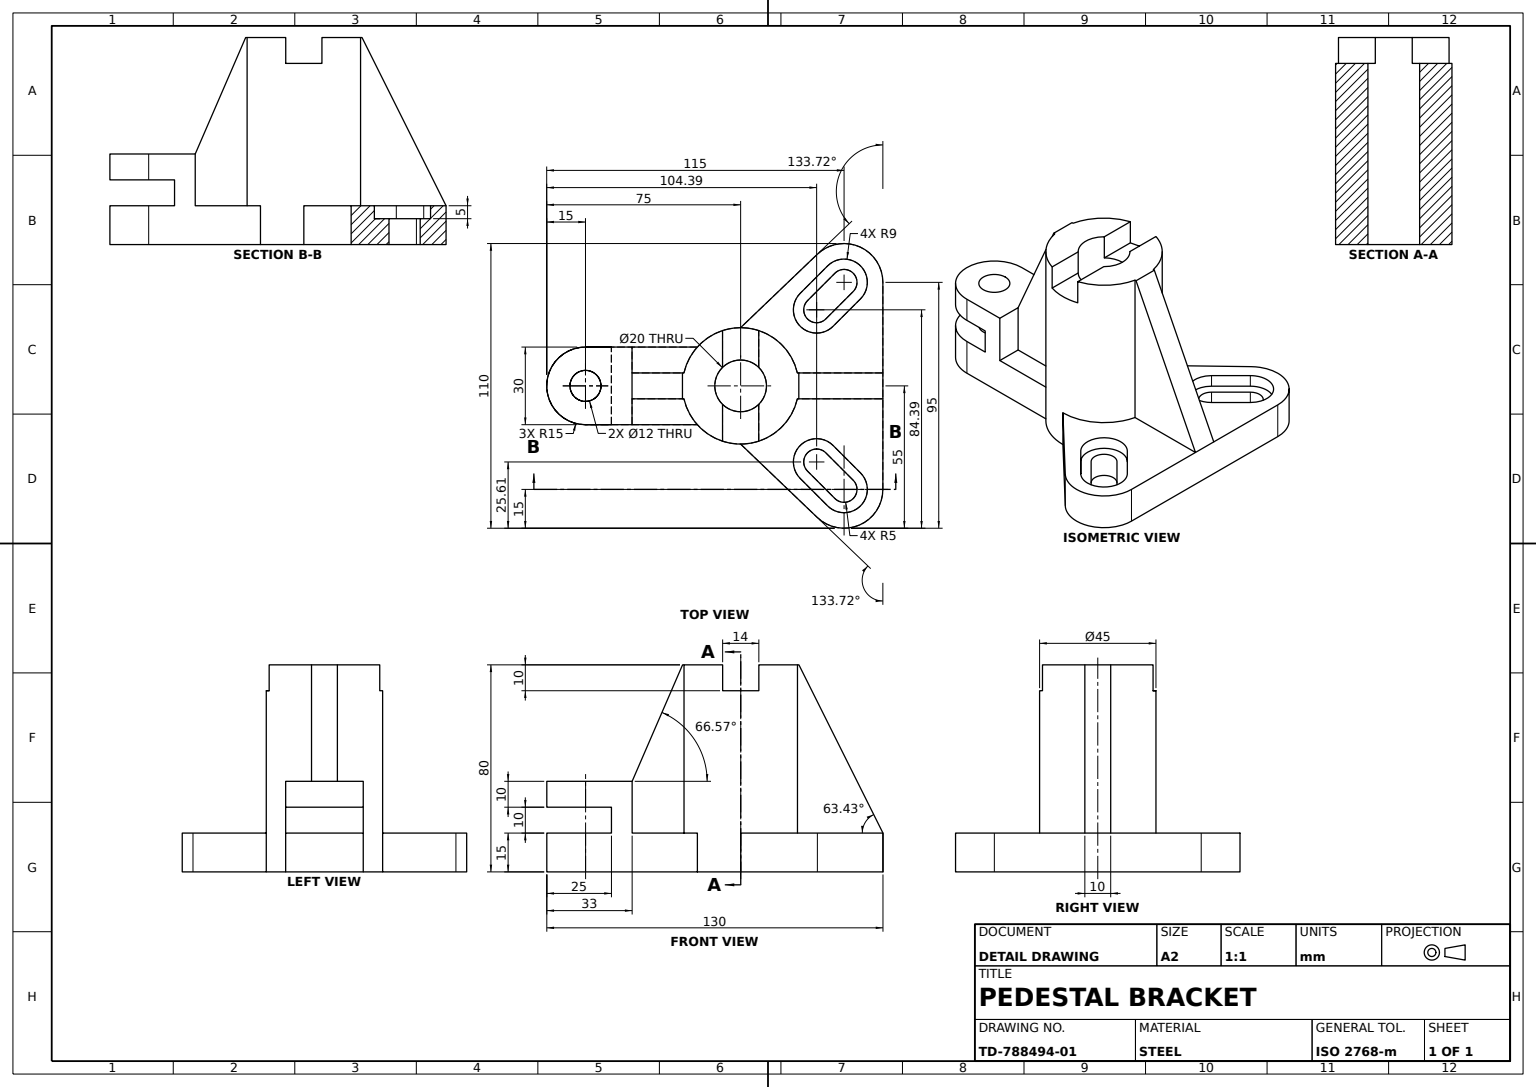
solid
v1 (-60,15,-6)
v2 (-60,15,6)
e1 v1 v2 CIRCLE(AX(P(-60,15,0),D(0,-1,0),D(0,0,-1)),6)
e2 v2 v1 CIRCLE(AX(P(-60,15,0),D(0,-1,0),D(0,0,-1)),6)
v3 (-60,15,15)
v4 (-60,15,-15)
e3 v3 v4 CIRCLE(AX(P(-60,15,0),D(0,-1,0),D(0,0,-1)),15)
v5 (-50,15,15)
e4 v5 v3 LINE
v6 (-50,15,-15)
e5 v5 v6 LINE
e6 v4 v6 LINE
face PLANE(AX(P(-75,15,15),D(0,-1,0),D(0,0,-1))) rev [e1 e2] [-e3 -e4 e5 -e6]
v7 (29.632367,15,-50.840304)
v8 (0,15,-22.5)
e7 v7 v8 LINE
v9 (29.632367,0,-50.840304)
e8 v7 v9 LINE
v10 (0,0,-22.5)
e9 v9 v10 LINE
e10 v8 v10 LINE
face PLANE(AX(P(-11.238829,15,-11.751219),D(0.691175529,0,0.722686923),D(0.722686923,0,-0.691175529))) rev [-e7 e8 e9 -e10]
v11 (36.464466,10,43.535534)
v12 (36.464466,0,43.535534)
e11 v11 v12 LINE
v13 (25.857864,0,32.928932)
e12 v12 v13 LINE
v14 (25.857864,10,32.928932)
e13 v14 v13 LINE
e14 v11 v14 LINE
face PLANE(AX(P(36.464466,80,43.535534),D(0.707106781,0,-0.707106781),D(-0.707106781,0,-0.707106781))) [e11 e12 -e13 -e14]
v15 (-42,35,-5)
v16 (-42,35,-15)
e15 v15 v16 LINE
v17 (-60,35,-15)
e16 v16 v17 LINE
v18 (-60,35,15)
e17 v17 v18 CIRCLE(AX(P(-60,35,0),D(0,1,0),D(0,0,1)),15)
v19 (-42,35,15)
e18 v18 v19 LINE
v20 (-42,35,5)
e19 v19 v20 LINE
e20 v15 v20 LINE
v21 (-60,35,6)
v22 (-60,35,-6)
e21 v21 v22 CIRCLE(AX(P(-60,35,0),D(0,1,0),D(0,0,1)),6)
e22 v22 v21 CIRCLE(AX(P(-60,35,0),D(0,1,0),D(0,0,1)),6)
face PLANE(AX(P(-60,35,0),D(0,1,0),D(0,0,1))) [e15 e16 e17 e18 e19 -e20] [-e21 -e22]
v23 (-16.77051,15,-15)
v24 (-21.937411,15,-5)
e23 v23 v24 CIRCLE(AX(P(0,15,0),D(0,1,0),D(0,0,1)),22.5)
v25 (-42,15,-15)
e24 v25 v23 LINE
v26 (-42,15,-5)
e25 v26 v25 LINE
e26 v26 v24 LINE
face PLANE(AX(P(0,15,0),D(0,1,0),D(0,0,1))) [-e23 -e24 -e25 e26]
v27 (-42,15,15)
v28 (-42,15,5)
e27 v27 v28 LINE
v29 (-16.77051,15,15)
e28 v27 v29 LINE
v30 (-21.937411,15,5)
e29 v30 v29 CIRCLE(AX(P(0,15,0),D(0,1,0),D(0,0,1)),22.5)
e30 v28 v30 LINE
face PLANE(AX(P(0,15,0),D(0,1,0),D(0,0,1))) [-e27 e28 -e29 -e30]
v31 (-21.937411,80,5)
v32 (-7,80,21.383405)
e31 v31 v32 CIRCLE(AX(P(0,80,0),D(0,1,0),D(0,0,1)),22.5)
e32 v31 v30 LINE
v33 (-16.77051,0,15)
e33 v29 v33 LINE
v34 (0,0,22.5)
e34 v33 v34 CIRCLE(AX(P(0,0,0),D(0,1,0),D(0,0,1)),22.5)
v35 (0,15,22.5)
e35 v35 v34 LINE
v36 (21.937411,15,5)
e36 v35 v36 CIRCLE(AX(P(0,15,0),D(0,1,0),D(0,0,1)),22.5)
v37 (21.937411,80,5)
e37 v36 v37 LINE
v38 (7,80,21.383405)
e38 v38 v37 CIRCLE(AX(P(0,80,0),D(0,1,0),D(0,0,1)),22.5)
v39 (7,70,21.383405)
e39 v38 v39 LINE
v40 (-7,70,21.383405)
e40 v40 v39 CIRCLE(AX(P(0,70,0),D(0,1,0),D(0,0,1)),22.5)
e41 v40 v32 LINE
face CYL(AX(P(0,80,0),D(0,-1,0),D(0,0,-1)),22.5) [-e31 e32 e29 e33 e34 -e35 e36 e37 -e38 e39 -e40 e41]
v41 (40,10,-45)
v42 (40,0,-45)
e42 v41 v42 LINE
v43 (36.464466,10,-43.535534)
e43 v43 v41 CIRCLE(AX(P(40,10,-40),D(0,-1,0),D(0,0,1)),5)
v44 (36.464466,0,-43.535534)
e44 v43 v44 LINE
e45 v44 v42 CIRCLE(AX(P(40,0,-40),D(0,-1,0),D(0,0,1)),5)
face CYL(AX(P(40,80,-40),D(0,-1,0),D(0,0,-1)),5) rev [-e42 -e43 e44 e45]
v45 (22.5,80,-5)
v46 (55,15,-5)
e46 v45 v46 LINE
v47 (21.937411,15,-5)
e47 v47 v46 LINE
v48 (21.937411,80,-5)
e48 v47 v48 LINE
e49 v48 v45 LINE
face PLANE(AX(P(-10,40,-5),D(0,0,1),D(1,0,0))) rev [e46 -e47 e48 e49]
v49 (46.363961,10,33.636039)
v50 (35.757359,10,23.029437)
e50 v49 v50 LINE
v51 (46.363961,15,33.636039)
e51 v49 v51 LINE
v52 (35.757359,15,23.029437)
e52 v51 v52 LINE
e53 v50 v52 LINE
face PLANE(AX(P(46.363961,10,33.636039),D(0.707106781,0,-0.707106781),D(-0.707106781,0,-0.707106781))) rev [-e50 e51 e52 -e53]
v53 (40,10,49)
v54 (40,15,49)
e54 v53 v54 LINE
e55 v54 v51 CIRCLE(AX(P(40,15,40),D(0,1,0),D(0,0,1)),9)
e56 v53 v49 CIRCLE(AX(P(40,10,40),D(0,1,0),D(0,0,1)),9)
face CYL(AX(P(40,10,40),D(0,1,0),D(0,0,1)),9) rev [e54 e55 -e51 -e56]
v55 (0,70,-22.5)
v56 (-7,70,-21.383405)
e57 v55 v56 CIRCLE(AX(P(0,70,0),D(0,1,0),D(0,0,1)),22.5)
e58 v55 v8 LINE
v57 (-16.77051,0,-15)
e59 v10 v57 CIRCLE(AX(P(0,0,0),D(0,1,0),D(0,0,1)),22.5)
e60 v23 v57 LINE
v58 (-21.937411,80,-5)
e61 v58 v24 LINE
v59 (-7,80,-21.383405)
e62 v59 v58 CIRCLE(AX(P(0,80,0),D(0,1,0),D(0,0,1)),22.5)
e63 v59 v56 LINE
face CYL(AX(P(0,80,0),D(0,-1,0),D(0,0,-1)),22.5) [-e57 e58 e10 e59 -e60 e23 -e61 -e62 e63]
v60 (29.393398,15,-20.393398)
v61 (35.757359,15,-23.029437)
e64 v60 v61 CIRCLE(AX(P(29.393398,15,-29.393398),D(0,1,0),D(0,0,1)),9)
v62 (35.757359,10,-23.029437)
e65 v62 v61 LINE
v63 (29.393398,10,-20.393398)
e66 v63 v62 CIRCLE(AX(P(29.393398,10,-29.393398),D(0,1,0),D(0,0,1)),9)
e67 v63 v60 LINE
face CYL(AX(P(29.393398,10,-29.393398),D(0,1,0),D(0,0,1)),9) rev [e64 -e65 -e66 e67]
v64 (-50,25,-15)
e68 v6 v64 LINE
v65 (-50,25,15)
e69 v65 v5 LINE
e70 v64 v65 LINE
face PLANE(AX(P(-50,0,0),D(1,0,0),D(0,0,-1))) rev [-e68 -e5 -e69 -e70]
v66 (46.363961,15,-33.636039)
v67 (33.636039,15,-46.363961)
e71 v66 v67 CIRCLE(AX(P(40,15,-40),D(0,1,0),D(0,0,1)),9)
v68 (33.636039,10,-46.363961)
e72 v68 v67 LINE
v69 (46.363961,10,-33.636039)
e73 v69 v68 CIRCLE(AX(P(40,10,-40),D(0,1,0),D(0,0,1)),9)
e74 v69 v66 LINE
face CYL(AX(P(40,10,-40),D(0,1,0),D(0,0,1)),9) rev [e71 -e72 -e73 e74]
v70 (-22.5,80,-5)
e75 v70 v15 LINE
e76 v58 v70 LINE
e77 v26 v15 LINE
face PLANE(AX(P(-10,40,-5),D(0,0,1),D(1,0,0))) rev [-e75 -e76 e61 -e26 e77]
v71 (43.535534,0,-36.464466)
v72 (32.928932,0,-25.857864)
e78 v71 v72 LINE
v73 (32.928932,10,-25.857864)
e79 v73 v72 LINE
v74 (43.535534,10,-36.464466)
e80 v74 v73 LINE
e81 v74 v71 LINE
face PLANE(AX(P(32.928932,80,-25.857864),D(-0.707106781,0,-0.707106781),D(-0.707106781,0,0.707106781))) [e78 -e79 -e80 e81]
v75 (33.636039,15,46.363961)
e82 v75 v54 CIRCLE(AX(P(40,15,40),D(0,1,0),D(0,0,1)),9)
v76 (33.636039,10,46.363961)
e83 v76 v53 CIRCLE(AX(P(40,10,40),D(0,1,0),D(0,0,1)),9)
e84 v76 v75 LINE
face CYL(AX(P(40,10,40),D(0,1,0),D(0,0,1)),9) rev [e82 -e54 -e83 e84]
v77 (32.928932,10,25.857864)
v78 (32.928932,0,25.857864)
e85 v77 v78 LINE
v79 (43.535534,0,36.464466)
e86 v78 v79 LINE
v80 (43.535534,10,36.464466)
e87 v80 v79 LINE
e88 v77 v80 LINE
face PLANE(AX(P(43.535534,80,36.464466),D(-0.707106781,0,0.707106781),D(0.707106781,0,0.707106781))) [e85 e86 -e87 -e88]
v81 (22.5,80,5)
e89 v37 v81 LINE
e90 v45 v81 LINE
v82 (7,80,-21.383405)
e91 v48 v82 CIRCLE(AX(P(0,80,0),D(0,1,0),D(0,0,1)),22.5)
v83 (7,80,-7.141428)
e92 v83 v82 LINE
v84 (7,80,7.141428)
e93 v84 v83 CIRCLE(AX(P(0,80,0),D(0,1,0),D(0,0,1)),10)
e94 v38 v84 LINE
face PLANE(AX(P(0,80,0),D(0,1,0),D(0,0,1))) [e89 -e90 -e49 e91 -e92 -e93 -e94 e38]
v85 (-60,25,-6)
e95 v85 v22 LINE
v86 (-60,25,6)
e96 v86 v85 CIRCLE(AX(P(-60,25,0),D(0,1,0),D(0,0,1)),6)
e97 v86 v21 LINE
face CYL(AX(P(-60,0,0),D(0,1,0),D(0,0,1)),6) rev [e21 -e95 -e96 e97]
v87 (-60,25,-15)
e98 v17 v87 LINE
v88 (-60,25,15)
e99 v87 v88 CIRCLE(AX(P(-60,25,0),D(0,1,0),D(0,0,1)),15)
e100 v18 v88 LINE
face CYL(AX(P(-60,15,0),D(0,-1,0),D(0,0,-1)),15) [e98 e99 -e100 -e17]
v89 (29.393398,10,24.393398)
e101 v89 v77 CIRCLE(AX(P(29.393398,10,29.393398),D(0,-1,0),D(0,0,1)),5)
v90 (29.393398,0,24.393398)
e102 v89 v90 LINE
e103 v90 v78 CIRCLE(AX(P(29.393398,0,29.393398),D(0,-1,0),D(0,0,1)),5)
face CYL(AX(P(29.393398,80,29.393398),D(0,-1,0),D(0,0,-1)),5) rev [-e101 e102 e103 -e85]
e104 v85 v86 CIRCLE(AX(P(-60,25,0),D(0,1,0),D(0,0,1)),6)
face CYL(AX(P(-60,0,0),D(0,1,0),D(0,0,1)),6) rev [-e97 -e104 e95 e22]
v91 (55,15,5)
e105 v91 v46 LINE
e106 v81 v91 LINE
face PLANE(AX(P(22.5,80,0),D(-0.894427191,-0.447213595,0),D(0.447213595,-0.894427191,0))) rev [e105 -e46 e90 e106]
v92 (23.029437,15,35.757359)
e107 v92 v75 LINE
v93 (23.029437,10,35.757359)
e108 v93 v76 LINE
e109 v93 v92 LINE
face PLANE(AX(P(33.636039,10,46.363961),D(-0.707106781,0,0.707106781),D(0.707106781,0,0.707106781))) rev [e107 -e84 -e108 e109]
v94 (0,70,10)
v95 (7,70,7.141428)
e110 v94 v95 CIRCLE(AX(P(0,70,0),D(0,1,0),D(0,0,1)),10)
v96 (-7,70,7.141428)
e111 v96 v94 CIRCLE(AX(P(0,70,0),D(0,1,0),D(0,0,1)),10)
e112 v96 v40 LINE
e113 v39 v95 LINE
face PLANE(AX(P(0,70,0),D(0,1,0),D(0,0,1))) [-e110 -e111 e112 e40 e113]
v97 (-7,80,-7.141428)
e114 v59 v97 LINE
v98 (-7,70,-7.141428)
e115 v98 v97 LINE
e116 v56 v98 LINE
face PLANE(AX(P(-7,70,-7.141428),D(-1,0,0),D(0,0,1))) rev [e114 -e115 -e116 -e63]
e117 v14 v89 CIRCLE(AX(P(29.393398,10,29.393398),D(0,-1,0),D(0,0,1)),5)
e118 v13 v90 CIRCLE(AX(P(29.393398,0,29.393398),D(0,-1,0),D(0,0,1)),5)
face CYL(AX(P(29.393398,80,29.393398),D(0,-1,0),D(0,0,-1)),5) rev [-e102 -e117 e13 e118]
e119 v19 v27 LINE
e120 v28 v20 LINE
face PLANE(AX(P(-42,35,-15),D(-1,0,0),D(0,0,1))) rev [e119 e27 e120 -e19]
v99 (23.029437,15,-35.757359)
e121 v99 v60 CIRCLE(AX(P(29.393398,15,-29.393398),D(0,1,0),D(0,0,1)),9)
e122 v67 v99 LINE
e123 v61 v66 LINE
e124 v47 v8 CIRCLE(AX(P(0,15,0),D(0,1,0),D(0,0,1)),22.5)
v100 (55,15,-40)
e125 v46 v100 LINE
v101 (40,15,-55)
e126 v100 v101 CIRCLE(AX(P(40,15,-40),D(0,1,0),D(0,0,1)),15)
e127 v101 v7 CIRCLE(AX(P(40,15,-40),D(0,1,0),D(0,0,1)),15)
face PLANE(AX(P(0,15,0),D(0,1,0),D(0,0,1))) [-e64 -e121 -e122 -e71 -e123] [-e124 e47 e125 e126 e127 e7]
v102 (7,70,-7.141428)
v103 (7,70,-21.383405)
e128 v102 v103 LINE
e129 v102 v83 LINE
e130 v103 v82 LINE
face PLANE(AX(P(7,70,-7.141428),D(1,0,0),D(0,0,-1))) rev [-e128 e129 e92 -e130]
e131 v16 v25 LINE
face PLANE(AX(P(-42,35,-15),D(-1,0,0),D(0,0,1))) rev [e25 -e131 -e15 -e77]
v104 (0,70,-10)
e132 v102 v104 CIRCLE(AX(P(0,70,0),D(0,1,0),D(0,0,1)),10)
v105 (0,0,-10)
e133 v105 v104 LINE
v106 (0,0,10)
e134 v106 v105 CIRCLE(AX(P(0,0,0),D(0,1,0),D(0,0,1)),10)
e135 v106 v94 LINE
e136 v95 v84 LINE
face CYL(AX(P(0,70,0),D(0,1,0),D(0,0,1)),10) rev [e132 -e133 -e134 e135 e110 e136 e93 -e129]
v107 (25.857864,0,-32.928932)
e137 v107 v44 LINE
v108 (25.857864,10,-32.928932)
e138 v108 v43 LINE
e139 v108 v107 LINE
face PLANE(AX(P(25.857864,80,-32.928932),D(0.707106781,0,0.707106781),D(0.707106781,0,-0.707106781))) [e137 -e44 -e138 e139]
v109 (-60,0,6)
v110 (-60,0,-6)
e140 v109 v110 CIRCLE(AX(P(-60,0,0),D(0,1,0),D(0,0,1)),6)
e141 v109 v2 LINE
e142 v110 v1 LINE
face CYL(AX(P(-60,0,0),D(0,1,0),D(0,0,1)),6) rev [-e140 e141 -e1 -e142]
e143 v88 v65 LINE
e144 v87 v64 LINE
face PLANE(AX(P(-75,25,15),D(0,1,0),D(0,0,1))) rev [e104 e96] [-e143 -e99 e144 e70]
e145 v103 v55 CIRCLE(AX(P(0,70,0),D(0,1,0),D(0,0,1)),22.5)
face CYL(AX(P(0,80,0),D(0,-1,0),D(0,0,-1)),22.5) [-e145 e130 -e91 -e48 e124 -e58]
e146 v41 v74 CIRCLE(AX(P(40,10,-40),D(0,-1,0),D(0,0,1)),5)
e147 v42 v71 CIRCLE(AX(P(40,0,-40),D(0,-1,0),D(0,0,1)),5)
face CYL(AX(P(40,80,-40),D(0,-1,0),D(0,0,-1)),5) rev [-e81 -e146 e42 e147]
e148 v104 v98 CIRCLE(AX(P(0,70,0),D(0,1,0),D(0,0,1)),10)
face PLANE(AX(P(0,70,0),D(0,1,0),D(0,0,1))) [e116 -e148 -e132 e128 e145 e57]
v111 (40,0,-55)
e149 v101 v111 LINE
e150 v111 v9 CIRCLE(AX(P(40,0,-40),D(0,1,0),D(0,0,1)),15)
face CYL(AX(P(40,15,-40),D(0,-1,0),D(0,0,-1)),15) [e149 e150 -e8 -e127]
v112 (-22.5,80,5)
e151 v112 v20 LINE
e152 v31 v112 LINE
face PLANE(AX(P(-10,40,5),D(0,0,1),D(1,0,0))) [e151 -e120 e30 -e32 e152]
e153 v70 v112 LINE
v113 (-7,80,7.141428)
e154 v113 v32 LINE
e155 v97 v113 CIRCLE(AX(P(0,80,0),D(0,1,0),D(0,0,1)),10)
face PLANE(AX(P(0,80,0),D(0,1,0),D(0,0,1))) [e62 e76 e153 -e152 e31 -e154 -e155 -e114]
e156 v110 v109 CIRCLE(AX(P(-60,0,0),D(0,1,0),D(0,0,1)),6)
face CYL(AX(P(-60,0,0),D(0,1,0),D(0,0,1)),6) rev [-e156 e142 -e2 -e141]
v114 (23.029437,10,-35.757359)
e157 v114 v63 CIRCLE(AX(P(29.393398,10,-29.393398),D(0,1,0),D(0,0,1)),9)
e158 v114 v99 LINE
face CYL(AX(P(29.393398,10,-29.393398),D(0,1,0),D(0,0,1)),9) rev [-e157 e158 e121 -e67]
v115 (29.632367,15,50.840304)
v116 (29.632367,0,50.840304)
e159 v115 v116 LINE
e160 v35 v115 LINE
e161 v34 v116 LINE
face PLANE(AX(P(-11.238829,15,11.751219),D(0.691175529,0,-0.722686923),D(-0.722686923,0,-0.691175529))) rev [-e159 -e160 e35 e161]
v117 (55,0,-40)
e162 v100 v117 LINE
e163 v117 v111 CIRCLE(AX(P(40,0,-40),D(0,1,0),D(0,0,1)),15)
face CYL(AX(P(40,15,-40),D(0,-1,0),D(0,0,-1)),15) [-e126 e162 e163 -e149]
e164 v80 v11 CIRCLE(AX(P(40,10,40),D(0,-1,0),D(0,0,1)),5)
e165 v50 v93 CIRCLE(AX(P(29.393398,10,29.393398),D(0,1,0),D(0,0,1)),9)
face PLANE(AX(P(40,10,40),D(0,1,0),D(0,0,1))) [e117 e101 e88 e164 e14] [e50 e165 e108 e83 e56]
v118 (-60,0,15)
e166 v3 v118 LINE
v119 (-60,0,-15)
e167 v4 v119 LINE
e168 v119 v118 CIRCLE(AX(P(-60,0,0),D(0,1,0),D(0,0,1)),15)
face CYL(AX(P(-60,15,0),D(0,-1,0),D(0,0,-1)),15) [-e166 e3 e167 e168]
face PLANE(AX(P(7,70,26.706406),D(1,0,0),D(0,0,-1))) rev [-e136 -e113 -e39 e94]
e169 v96 v113 LINE
e170 v105 v106 CIRCLE(AX(P(0,0,0),D(0,1,0),D(0,0,1)),10)
face CYL(AX(P(0,70,0),D(0,1,0),D(0,0,1)),10) rev [e155 -e169 e111 -e135 -e170 e133 e148 e115]
e171 v119 v57 LINE
face PLANE(AX(P(0,15,-15),D(0,0,-1),D(-1,0,0))) [e68 -e144 -e98 -e16 e131 e24 e60 -e171 -e167 e6]
e172 v72 v107 CIRCLE(AX(P(29.393398,0,-29.393398),D(0,-1,0),D(0,0,1)),5)
e173 v73 v108 CIRCLE(AX(P(29.393398,10,-29.393398),D(0,-1,0),D(0,0,1)),5)
face CYL(AX(P(29.393398,80,-29.393398),D(0,-1,0),D(0,0,-1)),5) rev [e172 -e139 -e173 e79]
e174 v79 v12 CIRCLE(AX(P(40,0,40),D(0,-1,0),D(0,0,1)),5)
face CYL(AX(P(40,80,40),D(0,-1,0),D(0,0,-1)),5) rev [e174 -e11 -e164 e87]
e175 v68 v114 LINE
face PLANE(AX(P(33.636039,10,-46.363961),D(-0.707106781,0,-0.707106781),D(-0.707106781,0,0.707106781))) rev [-e175 e72 e122 -e158]
e176 v62 v69 LINE
face PLANE(AX(P(40,10,-40),D(0,1,0),D(0,0,1))) [e157 e66 e176 e73 e175] [e43 e146 e80 e173 e138]
e177 v118 v33 LINE
v120 (55,0,40)
e178 v120 v117 LINE
e179 v116 v120 CIRCLE(AX(P(40,0,40),D(0,1,0),D(0,0,1)),15)
face PLANE(AX(P(0,0,0),D(0,1,0),D(0,0,1))) rev [-e86 -e103 -e118 -e12 -e174] [-e161 -e34 -e177 -e168 e171 -e59 -e9 -e150 -e163 -e178 -e179] [-e45 -e137 -e172 -e78 -e147] [e140 e156] [e134 e170]
e180 v52 v92 CIRCLE(AX(P(29.393398,15,29.393398),D(0,1,0),D(0,0,1)),9)
e181 v36 v91 LINE
v121 (55,15,40)
e182 v115 v121 CIRCLE(AX(P(40,15,40),D(0,1,0),D(0,0,1)),15)
e183 v121 v91 LINE
face PLANE(AX(P(0,15,0),D(0,1,0),D(0,0,1))) [-e55 -e82 -e107 -e180 -e52] [-e181 -e36 e160 e182 e183]
e184 v121 v120 LINE
face PLANE(AX(P(55,15,0),D(-1,0,0),D(0,0,1))) rev [-e162 -e125 -e105 -e183 e184 e178]
face PLANE(AX(P(-10,40,5),D(0,0,1),D(1,0,0))) [-e37 e181 -e106 -e89]
face PLANE(AX(P(46.363961,10,-33.636039),D(0.707106781,0,0.707106781),D(0.707106781,0,-0.707106781))) rev [e123 -e74 -e176 e65]
face CYL(AX(P(40,15,40),D(0,-1,0),D(0,0,-1)),15) [-e182 e159 e179 -e184]
face PLANE(AX(P(-7,70,26.706406),D(-1,0,0),D(0,0,1))) rev [-e112 e169 e154 -e41]
face PLANE(AX(P(0,15,15),D(0,0,-1),D(-1,0,0))) rev [e166 e177 -e33 -e28 -e119 -e18 e100 e143 e69 e4]
face PLANE(AX(P(-22.5,80,0),D(-0.917555625,0.397607438,0),D(-0.397607438,-0.917555625,0))) [e20 -e151 -e153 e75]
face CYL(AX(P(29.393398,10,29.393398),D(0,1,0),D(0,0,1)),9) rev [e53 e180 -e109 -e165]
